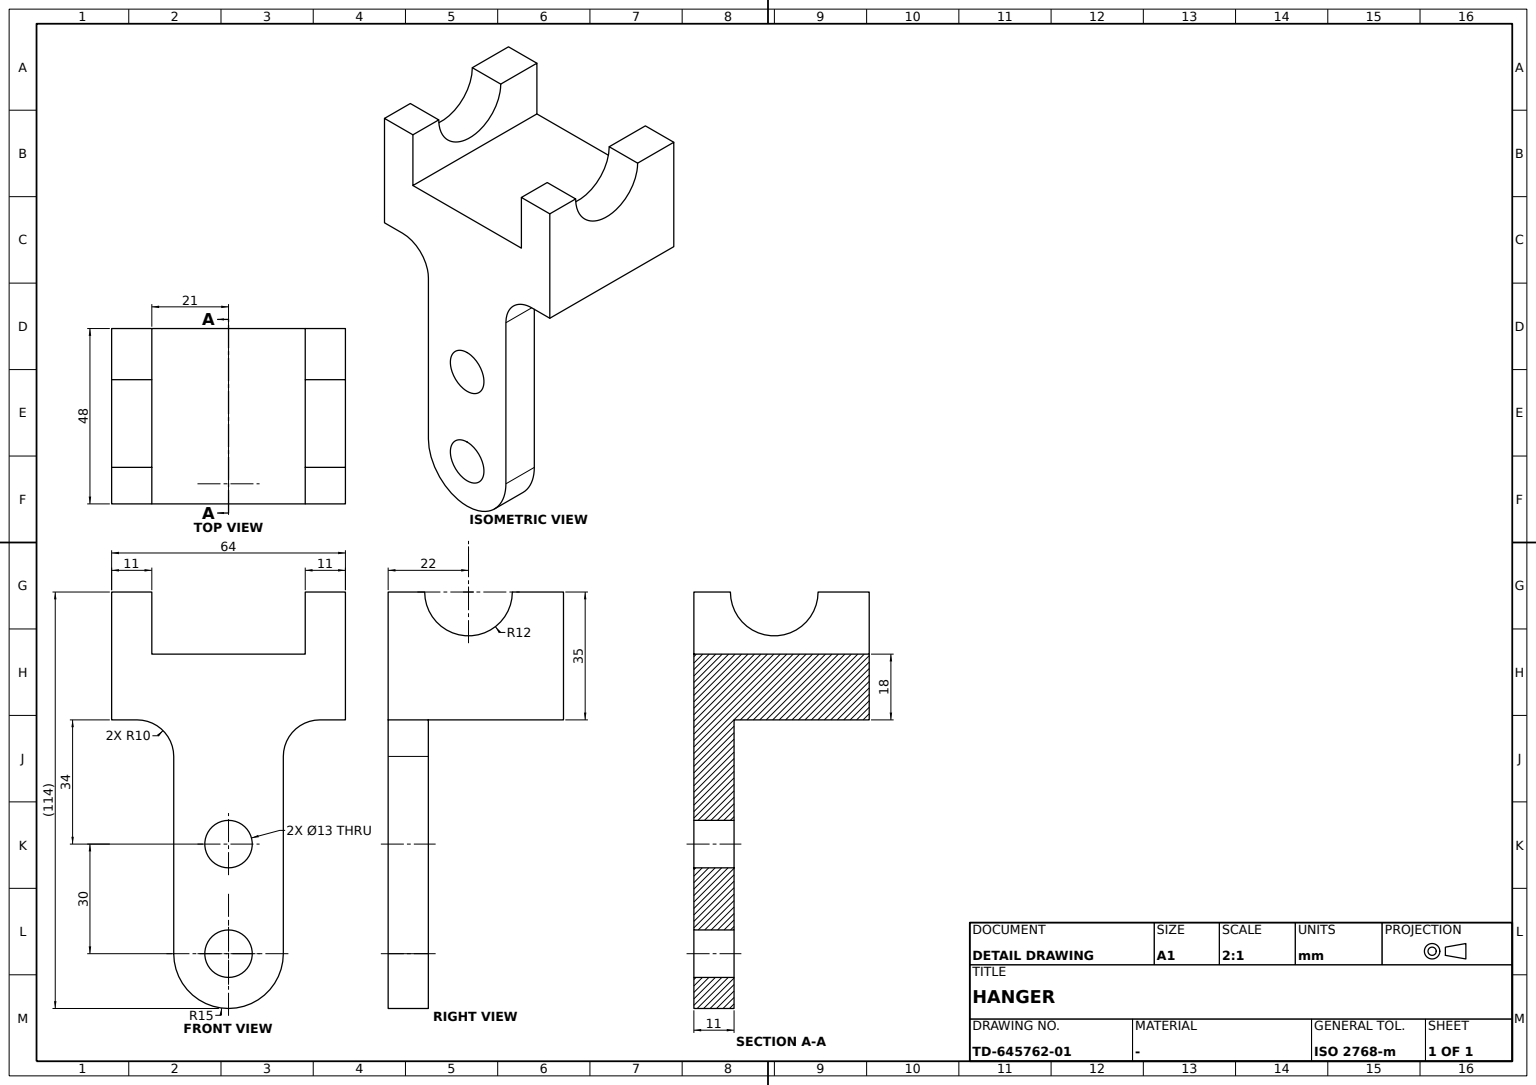
ISO-10303-21;
HEADER;
FILE_DESCRIPTION((''),'2;1');
FILE_NAME('','',(''),(''),'','','');
FILE_SCHEMA(('AUTOMOTIVE_DESIGN'));
ENDSEC;
DATA;
#1=APPLICATION_CONTEXT('');
#2=PRODUCT_CONTEXT('',#1,'mechanical');
#3=PRODUCT('','','',(#2));
#4=PRODUCT_DEFINITION_FORMATION('','',#3);
#5=PRODUCT_DEFINITION_CONTEXT('',#1,'design');
#6=PRODUCT_DEFINITION('','',#4,#5);
#7=PRODUCT_DEFINITION_SHAPE('','',#6);
#8=(LENGTH_UNIT()NAMED_UNIT(*)SI_UNIT(.MILLI.,.METRE.));
#9=(NAMED_UNIT(*)PLANE_ANGLE_UNIT()SI_UNIT($,.RADIAN.));
#10=(NAMED_UNIT(*)SI_UNIT($,.STERADIAN.)SOLID_ANGLE_UNIT());
#11=UNCERTAINTY_MEASURE_WITH_UNIT(LENGTH_MEASURE(0.005),#8,'distance_accuracy_value','');
#12=(GEOMETRIC_REPRESENTATION_CONTEXT(3)GLOBAL_UNCERTAINTY_ASSIGNED_CONTEXT((#11))GLOBAL_UNIT_ASSIGNED_CONTEXT((#8,#9,#10))REPRESENTATION_CONTEXT('',''));
#13=CARTESIAN_POINT('',(32.,48.,99.));
#14=VERTEX_POINT('',#13);
#15=CARTESIAN_POINT('',(32.,34.,99.));
#16=VERTEX_POINT('',#15);
#17=DIRECTION('',(0.,-1.,0.));
#18=VECTOR('',#17,1000.);
#19=LINE('',#13,#18);
#20=EDGE_CURVE('',#14,#16,#19,.T.);
#21=ORIENTED_EDGE('',*,*,#20,.F.);
#22=CARTESIAN_POINT('',(21.,48.,99.));
#23=VERTEX_POINT('',#22);
#24=DIRECTION('',(1.,0.,0.));
#25=VECTOR('',#24,1000.);
#26=LINE('',#22,#25);
#27=EDGE_CURVE('',#23,#14,#26,.T.);
#28=ORIENTED_EDGE('',*,*,#27,.F.);
#29=CARTESIAN_POINT('',(21.,34.,99.));
#30=VERTEX_POINT('',#29);
#31=LINE('',#22,#18);
#32=EDGE_CURVE('',#23,#30,#31,.T.);
#33=ORIENTED_EDGE('',*,*,#32,.T.);
#34=CARTESIAN_POINT('',(35.,34.,99.));
#35=LINE('',#34,#25);
#36=EDGE_CURVE('',#30,#16,#35,.T.);
#37=ORIENTED_EDGE('',*,*,#36,.T.);
#38=EDGE_LOOP('',(#21,#28,#33,#37));
#39=FACE_BOUND('',#38,.T.);
#40=DIRECTION('',(0.,0.,-1.));
#41=DIRECTION('',(-1.,0.,0.));
#42=AXIS2_PLACEMENT_3D('',#22,#40,#41);
#43=PLANE('',#42);
#44=ADVANCED_FACE('',(#39),#43,.F.);
#45=CARTESIAN_POINT('',(21.,48.,82.));
#46=VERTEX_POINT('',#45);
#47=CARTESIAN_POINT('',(21.,0.,82.));
#48=VERTEX_POINT('',#47);
#49=LINE('',#45,#18);
#50=EDGE_CURVE('',#46,#48,#49,.T.);
#51=ORIENTED_EDGE('',*,*,#50,.F.);
#52=CARTESIAN_POINT('',(-21.,48.,82.));
#53=VERTEX_POINT('',#52);
#54=LINE('',#52,#25);
#55=EDGE_CURVE('',#53,#46,#54,.T.);
#56=ORIENTED_EDGE('',*,*,#55,.F.);
#57=CARTESIAN_POINT('',(-21.,0.,82.));
#58=VERTEX_POINT('',#57);
#59=LINE('',#52,#18);
#60=EDGE_CURVE('',#53,#58,#59,.T.);
#61=ORIENTED_EDGE('',*,*,#60,.T.);
#62=LINE('',#57,#25);
#63=EDGE_CURVE('',#58,#48,#62,.T.);
#64=ORIENTED_EDGE('',*,*,#63,.T.);
#65=EDGE_LOOP('',(#51,#56,#61,#64));
#66=FACE_BOUND('',#65,.T.);
#67=AXIS2_PLACEMENT_3D('',#52,#40,#41);
#68=PLANE('',#67);
#69=ADVANCED_FACE('',(#66),#68,.F.);
#70=CARTESIAN_POINT('',(32.,10.,99.));
#71=VERTEX_POINT('',#70);
#72=CARTESIAN_POINT('',(32.,22.,99.));
#73=DIRECTION('',(0.,0.,1.));
#74=AXIS2_PLACEMENT_3D('',#72,#24,#73);
#75=CIRCLE('',#74,12.);
#76=EDGE_CURVE('',#71,#16,#75,.T.);
#77=ORIENTED_EDGE('',*,*,#76,.T.);
#78=ORIENTED_EDGE('',*,*,#36,.F.);
#79=CARTESIAN_POINT('',(21.,10.,99.));
#80=VERTEX_POINT('',#79);
#81=CARTESIAN_POINT('',(21.,22.,99.));
#82=AXIS2_PLACEMENT_3D('',#81,#41,#40);
#83=CIRCLE('',#82,12.);
#84=EDGE_CURVE('',#30,#80,#83,.T.);
#85=ORIENTED_EDGE('',*,*,#84,.T.);
#86=CARTESIAN_POINT('',(35.,10.,99.));
#87=VECTOR('',#41,1000.);
#88=LINE('',#86,#87);
#89=EDGE_CURVE('',#71,#80,#88,.T.);
#90=ORIENTED_EDGE('',*,*,#89,.F.);
#91=EDGE_LOOP('',(#77,#78,#85,#90));
#92=FACE_BOUND('',#91,.T.);
#93=CARTESIAN_POINT('',(35.,22.,99.));
#94=AXIS2_PLACEMENT_3D('',#93,#41,#73);
#95=CYLINDRICAL_SURFACE('',#94,12.);
#96=ADVANCED_FACE('',(#92),#95,.F.);
#97=CARTESIAN_POINT('',(-21.,10.,99.));
#98=VERTEX_POINT('',#97);
#99=CARTESIAN_POINT('',(-21.,0.,99.));
#100=VERTEX_POINT('',#99);
#101=CARTESIAN_POINT('',(-21.,48.,99.));
#102=LINE('',#101,#18);
#103=EDGE_CURVE('',#98,#100,#102,.T.);
#104=ORIENTED_EDGE('',*,*,#103,.F.);
#105=CARTESIAN_POINT('',(-32.,10.,99.));
#106=VERTEX_POINT('',#105);
#107=EDGE_CURVE('',#98,#106,#88,.T.);
#108=ORIENTED_EDGE('',*,*,#107,.T.);
#109=CARTESIAN_POINT('',(-32.,0.,99.));
#110=VERTEX_POINT('',#109);
#111=CARTESIAN_POINT('',(-32.,48.,99.));
#112=LINE('',#111,#18);
#113=EDGE_CURVE('',#106,#110,#112,.T.);
#114=ORIENTED_EDGE('',*,*,#113,.T.);
#115=LINE('',#109,#25);
#116=EDGE_CURVE('',#110,#100,#115,.T.);
#117=ORIENTED_EDGE('',*,*,#116,.T.);
#118=EDGE_LOOP('',(#104,#108,#114,#117));
#119=FACE_BOUND('',#118,.T.);
#120=AXIS2_PLACEMENT_3D('',#111,#40,#41);
#121=PLANE('',#120);
#122=ADVANCED_FACE('',(#119),#121,.F.);
#123=CARTESIAN_POINT('',(-21.,34.,99.));
#124=VERTEX_POINT('',#123);
#125=CARTESIAN_POINT('',(-21.,22.,99.));
#126=AXIS2_PLACEMENT_3D('',#125,#24,#73);
#127=CIRCLE('',#126,12.);
#128=EDGE_CURVE('',#98,#124,#127,.T.);
#129=ORIENTED_EDGE('',*,*,#128,.T.);
#130=CARTESIAN_POINT('',(-32.,34.,99.));
#131=VERTEX_POINT('',#130);
#132=EDGE_CURVE('',#131,#124,#35,.T.);
#133=ORIENTED_EDGE('',*,*,#132,.F.);
#134=CARTESIAN_POINT('',(-32.,22.,99.));
#135=AXIS2_PLACEMENT_3D('',#134,#41,#40);
#136=CIRCLE('',#135,12.);
#137=EDGE_CURVE('',#131,#106,#136,.T.);
#138=ORIENTED_EDGE('',*,*,#137,.T.);
#139=ORIENTED_EDGE('',*,*,#107,.F.);
#140=EDGE_LOOP('',(#129,#133,#138,#139));
#141=FACE_BOUND('',#140,.T.);
#142=ADVANCED_FACE('',(#141),#95,.F.);
#143=CARTESIAN_POINT('',(-25.,11.,64.));
#144=VERTEX_POINT('',#143);
#145=CARTESIAN_POINT('',(-25.,0.,64.));
#146=VERTEX_POINT('',#145);
#147=LINE('',#143,#18);
#148=EDGE_CURVE('',#144,#146,#147,.T.);
#149=ORIENTED_EDGE('',*,*,#148,.T.);
#150=CARTESIAN_POINT('',(-32.,0.,64.));
#151=VERTEX_POINT('',#150);
#152=CARTESIAN_POINT('',(32.,0.,64.));
#153=LINE('',#152,#87);
#154=EDGE_CURVE('',#146,#151,#153,.T.);
#155=ORIENTED_EDGE('',*,*,#154,.T.);
#156=CARTESIAN_POINT('',(-32.,48.,64.));
#157=VERTEX_POINT('',#156);
#158=LINE('',#156,#18);
#159=EDGE_CURVE('',#157,#151,#158,.T.);
#160=ORIENTED_EDGE('',*,*,#159,.F.);
#161=CARTESIAN_POINT('',(32.,48.,64.));
#162=VERTEX_POINT('',#161);
#163=LINE('',#161,#87);
#164=EDGE_CURVE('',#162,#157,#163,.T.);
#165=ORIENTED_EDGE('',*,*,#164,.F.);
#166=VERTEX_POINT('',#152);
#167=LINE('',#161,#18);
#168=EDGE_CURVE('',#162,#166,#167,.T.);
#169=ORIENTED_EDGE('',*,*,#168,.T.);
#170=CARTESIAN_POINT('',(25.,0.,64.));
#171=VERTEX_POINT('',#170);
#172=EDGE_CURVE('',#166,#171,#153,.T.);
#173=ORIENTED_EDGE('',*,*,#172,.T.);
#174=CARTESIAN_POINT('',(25.,11.,64.));
#175=VERTEX_POINT('',#174);
#176=LINE('',#174,#18);
#177=EDGE_CURVE('',#175,#171,#176,.T.);
#178=ORIENTED_EDGE('',*,*,#177,.F.);
#179=LINE('',#174,#87);
#180=EDGE_CURVE('',#175,#144,#179,.T.);
#181=ORIENTED_EDGE('',*,*,#180,.T.);
#182=EDGE_LOOP('',(#149,#155,#160,#165,#169,#173,#178,#181));
#183=FACE_BOUND('',#182,.T.);
#184=AXIS2_PLACEMENT_3D('',#161,#73,#24);
#185=PLANE('',#184);
#186=ADVANCED_FACE('',(#183),#185,.F.);
#187=CARTESIAN_POINT('',(0.,11.,36.5));
#188=VERTEX_POINT('',#187);
#189=CARTESIAN_POINT('',(0.,11.,23.5));
#190=VERTEX_POINT('',#189);
#191=CARTESIAN_POINT('',(0.,11.,30.));
#192=AXIS2_PLACEMENT_3D('',#191,#17,#24);
#193=CIRCLE('',#192,6.5);
#194=EDGE_CURVE('',#188,#190,#193,.T.);
#195=ORIENTED_EDGE('',*,*,#194,.F.);
#196=CARTESIAN_POINT('',(0.,0.,36.5));
#197=VERTEX_POINT('',#196);
#198=LINE('',#187,#18);
#199=EDGE_CURVE('',#197,#188,#198,.F.);
#200=ORIENTED_EDGE('',*,*,#199,.F.);
#201=CARTESIAN_POINT('',(0.,0.,23.5));
#202=VERTEX_POINT('',#201);
#203=CARTESIAN_POINT('',(0.,0.,30.));
#204=AXIS2_PLACEMENT_3D('',#203,#17,#24);
#205=CIRCLE('',#204,6.5);
#206=EDGE_CURVE('',#197,#202,#205,.T.);
#207=ORIENTED_EDGE('',*,*,#206,.T.);
#208=LINE('',#189,#18);
#209=EDGE_CURVE('',#190,#202,#208,.T.);
#210=ORIENTED_EDGE('',*,*,#209,.F.);
#211=EDGE_LOOP('',(#195,#200,#207,#210));
#212=FACE_BOUND('',#211,.T.);
#213=AXIS2_PLACEMENT_3D('',#191,#17,#40);
#214=CYLINDRICAL_SURFACE('',#213,6.5);
#215=ADVANCED_FACE('',(#212),#214,.F.);
#216=VERTEX_POINT('',#111);
#217=EDGE_CURVE('',#216,#131,#112,.T.);
#218=ORIENTED_EDGE('',*,*,#217,.T.);
#219=ORIENTED_EDGE('',*,*,#132,.T.);
#220=VERTEX_POINT('',#101);
#221=EDGE_CURVE('',#220,#124,#102,.T.);
#222=ORIENTED_EDGE('',*,*,#221,.F.);
#223=LINE('',#111,#25);
#224=EDGE_CURVE('',#216,#220,#223,.T.);
#225=ORIENTED_EDGE('',*,*,#224,.F.);
#226=EDGE_LOOP('',(#218,#219,#222,#225));
#227=FACE_BOUND('',#226,.T.);
#228=ADVANCED_FACE('',(#227),#121,.F.);
#229=ORIENTED_EDGE('',*,*,#55,.T.);
#230=VECTOR('',#73,1000.);
#231=LINE('',#45,#230);
#232=EDGE_CURVE('',#46,#23,#231,.T.);
#233=ORIENTED_EDGE('',*,*,#232,.T.);
#234=ORIENTED_EDGE('',*,*,#27,.T.);
#235=VECTOR('',#40,1000.);
#236=LINE('',#13,#235);
#237=EDGE_CURVE('',#14,#162,#236,.T.);
#238=ORIENTED_EDGE('',*,*,#237,.T.);
#239=ORIENTED_EDGE('',*,*,#164,.T.);
#240=LINE('',#156,#230);
#241=EDGE_CURVE('',#157,#216,#240,.T.);
#242=ORIENTED_EDGE('',*,*,#241,.T.);
#243=ORIENTED_EDGE('',*,*,#224,.T.);
#244=LINE('',#101,#235);
#245=EDGE_CURVE('',#220,#53,#244,.T.);
#246=ORIENTED_EDGE('',*,*,#245,.T.);
#247=EDGE_LOOP('',(#229,#233,#234,#238,#239,#242,#243,#246));
#248=FACE_BOUND('',#247,.T.);
#249=CARTESIAN_POINT('',(0.,48.,0.));
#250=AXIS2_PLACEMENT_3D('',#249,#17,#40);
#251=PLANE('',#250);
#252=ADVANCED_FACE('',(#248),#251,.F.);
#253=ORIENTED_EDGE('',*,*,#241,.F.);
#254=ORIENTED_EDGE('',*,*,#159,.T.);
#255=LINE('',#150,#230);
#256=EDGE_CURVE('',#151,#110,#255,.T.);
#257=ORIENTED_EDGE('',*,*,#256,.T.);
#258=ORIENTED_EDGE('',*,*,#113,.F.);
#259=ORIENTED_EDGE('',*,*,#137,.F.);
#260=ORIENTED_EDGE('',*,*,#217,.F.);
#261=EDGE_LOOP('',(#253,#254,#257,#258,#259,#260));
#262=FACE_BOUND('',#261,.T.);
#263=AXIS2_PLACEMENT_3D('',#156,#24,#40);
#264=PLANE('',#263);
#265=ADVANCED_FACE('',(#262),#264,.F.);
#266=CARTESIAN_POINT('',(15.,11.,0.));
#267=VERTEX_POINT('',#266);
#268=CARTESIAN_POINT('',(15.,11.,54.));
#269=VERTEX_POINT('',#268);
#270=LINE('',#266,#230);
#271=EDGE_CURVE('',#267,#269,#270,.T.);
#272=ORIENTED_EDGE('',*,*,#271,.T.);
#273=CARTESIAN_POINT('',(15.,0.,54.));
#274=VERTEX_POINT('',#273);
#275=LINE('',#268,#18);
#276=EDGE_CURVE('',#269,#274,#275,.T.);
#277=ORIENTED_EDGE('',*,*,#276,.T.);
#278=CARTESIAN_POINT('',(15.,0.,0.));
#279=VERTEX_POINT('',#278);
#280=LINE('',#278,#230);
#281=EDGE_CURVE('',#279,#274,#280,.T.);
#282=ORIENTED_EDGE('',*,*,#281,.F.);
#283=LINE('',#266,#18);
#284=EDGE_CURVE('',#267,#279,#283,.T.);
#285=ORIENTED_EDGE('',*,*,#284,.F.);
#286=EDGE_LOOP('',(#272,#277,#282,#285));
#287=FACE_BOUND('',#286,.T.);
#288=AXIS2_PLACEMENT_3D('',#266,#24,#40);
#289=PLANE('',#288);
#290=ADVANCED_FACE('',(#287),#289,.T.);
#291=EDGE_CURVE('',#190,#188,#193,.T.);
#292=ORIENTED_EDGE('',*,*,#291,.T.);
#293=ORIENTED_EDGE('',*,*,#194,.T.);
#294=EDGE_LOOP('',(#292,#293));
#295=FACE_BOUND('',#294,.T.);
#296=CARTESIAN_POINT('',(0.,11.,6.5));
#297=VERTEX_POINT('',#296);
#298=CARTESIAN_POINT('',(0.,11.,-6.5));
#299=VERTEX_POINT('',#298);
#300=CARTESIAN_POINT('',(0.,11.,0.));
#301=AXIS2_PLACEMENT_3D('',#300,#17,#24);
#302=CIRCLE('',#301,6.5);
#303=EDGE_CURVE('',#297,#299,#302,.T.);
#304=ORIENTED_EDGE('',*,*,#303,.T.);
#305=EDGE_CURVE('',#299,#297,#302,.T.);
#306=ORIENTED_EDGE('',*,*,#305,.T.);
#307=EDGE_LOOP('',(#304,#306));
#308=FACE_BOUND('',#307,.T.);
#309=CARTESIAN_POINT('',(0.,11.,-15.));
#310=VERTEX_POINT('',#309);
#311=CIRCLE('',#301,15.);
#312=EDGE_CURVE('',#310,#267,#311,.T.);
#313=ORIENTED_EDGE('',*,*,#312,.F.);
#314=CARTESIAN_POINT('',(-15.,11.,0.));
#315=VERTEX_POINT('',#314);
#316=EDGE_CURVE('',#315,#310,#311,.T.);
#317=ORIENTED_EDGE('',*,*,#316,.F.);
#318=CARTESIAN_POINT('',(-15.,11.,54.));
#319=VERTEX_POINT('',#318);
#320=LINE('',#318,#235);
#321=EDGE_CURVE('',#319,#315,#320,.T.);
#322=ORIENTED_EDGE('',*,*,#321,.F.);
#323=CARTESIAN_POINT('',(-25.,11.,54.));
#324=DIRECTION('',(0.,1.,0.));
#325=AXIS2_PLACEMENT_3D('',#323,#324,#24);
#326=CIRCLE('',#325,10.);
#327=EDGE_CURVE('',#144,#319,#326,.T.);
#328=ORIENTED_EDGE('',*,*,#327,.F.);
#329=ORIENTED_EDGE('',*,*,#180,.F.);
#330=CARTESIAN_POINT('',(25.,11.,54.));
#331=AXIS2_PLACEMENT_3D('',#330,#324,#24);
#332=CIRCLE('',#331,10.);
#333=EDGE_CURVE('',#269,#175,#332,.T.);
#334=ORIENTED_EDGE('',*,*,#333,.F.);
#335=ORIENTED_EDGE('',*,*,#271,.F.);
#336=EDGE_LOOP('',(#313,#317,#322,#328,#329,#334,#335));
#337=FACE_BOUND('',#336,.T.);
#338=AXIS2_PLACEMENT_3D('',#323,#324,#73);
#339=PLANE('',#338);
#340=ADVANCED_FACE('',(#295,#308,#337),#339,.T.);
#341=CARTESIAN_POINT('',(0.,0.,-15.));
#342=VERTEX_POINT('',#341);
#343=LINE('',#309,#18);
#344=EDGE_CURVE('',#310,#342,#343,.T.);
#345=ORIENTED_EDGE('',*,*,#344,.F.);
#346=ORIENTED_EDGE('',*,*,#312,.T.);
#347=ORIENTED_EDGE('',*,*,#284,.T.);
#348=CARTESIAN_POINT('',(0.,0.,0.));
#349=AXIS2_PLACEMENT_3D('',#348,#17,#24);
#350=CIRCLE('',#349,15.);
#351=EDGE_CURVE('',#342,#279,#350,.T.);
#352=ORIENTED_EDGE('',*,*,#351,.F.);
#353=EDGE_LOOP('',(#345,#346,#347,#352));
#354=FACE_BOUND('',#353,.T.);
#355=AXIS2_PLACEMENT_3D('',#300,#17,#40);
#356=CYLINDRICAL_SURFACE('',#355,15.);
#357=ADVANCED_FACE('',(#354),#356,.T.);
#358=CARTESIAN_POINT('',(0.,0.,6.5));
#359=VERTEX_POINT('',#358);
#360=CARTESIAN_POINT('',(0.,0.,-6.5));
#361=VERTEX_POINT('',#360);
#362=CIRCLE('',#349,6.5);
#363=EDGE_CURVE('',#359,#361,#362,.T.);
#364=ORIENTED_EDGE('',*,*,#363,.F.);
#365=EDGE_CURVE('',#361,#359,#362,.T.);
#366=ORIENTED_EDGE('',*,*,#365,.F.);
#367=EDGE_LOOP('',(#364,#366));
#368=FACE_BOUND('',#367,.T.);
#369=CARTESIAN_POINT('',(-15.,0.,54.));
#370=VERTEX_POINT('',#369);
#371=CARTESIAN_POINT('',(-25.,0.,54.));
#372=AXIS2_PLACEMENT_3D('',#371,#324,#24);
#373=CIRCLE('',#372,10.);
#374=EDGE_CURVE('',#146,#370,#373,.T.);
#375=ORIENTED_EDGE('',*,*,#374,.T.);
#376=CARTESIAN_POINT('',(-15.,0.,0.));
#377=VERTEX_POINT('',#376);
#378=LINE('',#369,#235);
#379=EDGE_CURVE('',#370,#377,#378,.T.);
#380=ORIENTED_EDGE('',*,*,#379,.T.);
#381=EDGE_CURVE('',#377,#342,#350,.T.);
#382=ORIENTED_EDGE('',*,*,#381,.T.);
#383=ORIENTED_EDGE('',*,*,#351,.T.);
#384=ORIENTED_EDGE('',*,*,#281,.T.);
#385=CARTESIAN_POINT('',(25.,0.,54.));
#386=AXIS2_PLACEMENT_3D('',#385,#324,#24);
#387=CIRCLE('',#386,10.);
#388=EDGE_CURVE('',#274,#171,#387,.T.);
#389=ORIENTED_EDGE('',*,*,#388,.T.);
#390=ORIENTED_EDGE('',*,*,#172,.F.);
#391=CARTESIAN_POINT('',(32.,0.,99.));
#392=VERTEX_POINT('',#391);
#393=LINE('',#391,#235);
#394=EDGE_CURVE('',#392,#166,#393,.T.);
#395=ORIENTED_EDGE('',*,*,#394,.F.);
#396=CARTESIAN_POINT('',(21.,0.,99.));
#397=VERTEX_POINT('',#396);
#398=LINE('',#396,#25);
#399=EDGE_CURVE('',#397,#392,#398,.T.);
#400=ORIENTED_EDGE('',*,*,#399,.F.);
#401=LINE('',#47,#230);
#402=EDGE_CURVE('',#48,#397,#401,.T.);
#403=ORIENTED_EDGE('',*,*,#402,.F.);
#404=ORIENTED_EDGE('',*,*,#63,.F.);
#405=LINE('',#99,#235);
#406=EDGE_CURVE('',#100,#58,#405,.T.);
#407=ORIENTED_EDGE('',*,*,#406,.F.);
#408=ORIENTED_EDGE('',*,*,#116,.F.);
#409=ORIENTED_EDGE('',*,*,#256,.F.);
#410=ORIENTED_EDGE('',*,*,#154,.F.);
#411=EDGE_LOOP('',(#375,#380,#382,#383,#384,#389,#390,#395,#400,#403,#404,#407,#408,#409,#410));
#412=FACE_BOUND('',#411,.T.);
#413=EDGE_CURVE('',#202,#197,#205,.T.);
#414=ORIENTED_EDGE('',*,*,#413,.F.);
#415=ORIENTED_EDGE('',*,*,#206,.F.);
#416=EDGE_LOOP('',(#414,#415));
#417=FACE_BOUND('',#416,.T.);
#418=AXIS2_PLACEMENT_3D('',#348,#17,#40);
#419=PLANE('',#418);
#420=ADVANCED_FACE('',(#368,#412,#417),#419,.T.);
#421=ORIENTED_EDGE('',*,*,#316,.T.);
#422=ORIENTED_EDGE('',*,*,#344,.T.);
#423=ORIENTED_EDGE('',*,*,#381,.F.);
#424=LINE('',#314,#18);
#425=EDGE_CURVE('',#315,#377,#424,.T.);
#426=ORIENTED_EDGE('',*,*,#425,.F.);
#427=EDGE_LOOP('',(#421,#422,#423,#426));
#428=FACE_BOUND('',#427,.T.);
#429=ADVANCED_FACE('',(#428),#356,.T.);
#430=LINE('',#298,#18);
#431=EDGE_CURVE('',#299,#361,#430,.T.);
#432=ORIENTED_EDGE('',*,*,#431,.T.);
#433=ORIENTED_EDGE('',*,*,#365,.T.);
#434=LINE('',#296,#18);
#435=EDGE_CURVE('',#359,#297,#434,.F.);
#436=ORIENTED_EDGE('',*,*,#435,.T.);
#437=ORIENTED_EDGE('',*,*,#305,.F.);
#438=EDGE_LOOP('',(#432,#433,#436,#437));
#439=FACE_BOUND('',#438,.T.);
#440=CYLINDRICAL_SURFACE('',#355,6.5);
#441=ADVANCED_FACE('',(#439),#440,.F.);
#442=ORIENTED_EDGE('',*,*,#89,.T.);
#443=EDGE_CURVE('',#80,#397,#31,.T.);
#444=ORIENTED_EDGE('',*,*,#443,.T.);
#445=ORIENTED_EDGE('',*,*,#399,.T.);
#446=EDGE_CURVE('',#71,#392,#19,.T.);
#447=ORIENTED_EDGE('',*,*,#446,.F.);
#448=EDGE_LOOP('',(#442,#444,#445,#447));
#449=FACE_BOUND('',#448,.T.);
#450=ADVANCED_FACE('',(#449),#43,.F.);
#451=ORIENTED_EDGE('',*,*,#425,.T.);
#452=ORIENTED_EDGE('',*,*,#379,.F.);
#453=LINE('',#318,#18);
#454=EDGE_CURVE('',#319,#370,#453,.T.);
#455=ORIENTED_EDGE('',*,*,#454,.F.);
#456=ORIENTED_EDGE('',*,*,#321,.T.);
#457=EDGE_LOOP('',(#451,#452,#455,#456));
#458=FACE_BOUND('',#457,.T.);
#459=AXIS2_PLACEMENT_3D('',#318,#41,#73);
#460=PLANE('',#459);
#461=ADVANCED_FACE('',(#458),#460,.T.);
#462=ORIENTED_EDGE('',*,*,#431,.F.);
#463=ORIENTED_EDGE('',*,*,#303,.F.);
#464=ORIENTED_EDGE('',*,*,#435,.F.);
#465=ORIENTED_EDGE('',*,*,#363,.T.);
#466=EDGE_LOOP('',(#462,#463,#464,#465));
#467=FACE_BOUND('',#466,.T.);
#468=ADVANCED_FACE('',(#467),#440,.F.);
#469=ORIENTED_EDGE('',*,*,#327,.T.);
#470=ORIENTED_EDGE('',*,*,#454,.T.);
#471=ORIENTED_EDGE('',*,*,#374,.F.);
#472=ORIENTED_EDGE('',*,*,#148,.F.);
#473=EDGE_LOOP('',(#469,#470,#471,#472));
#474=FACE_BOUND('',#473,.T.);
#475=AXIS2_PLACEMENT_3D('',#323,#17,#40);
#476=CYLINDRICAL_SURFACE('',#475,10.);
#477=ADVANCED_FACE('',(#474),#476,.F.);
#478=ORIENTED_EDGE('',*,*,#221,.T.);
#479=ORIENTED_EDGE('',*,*,#128,.F.);
#480=ORIENTED_EDGE('',*,*,#103,.T.);
#481=ORIENTED_EDGE('',*,*,#406,.T.);
#482=ORIENTED_EDGE('',*,*,#60,.F.);
#483=ORIENTED_EDGE('',*,*,#245,.F.);
#484=EDGE_LOOP('',(#478,#479,#480,#481,#482,#483));
#485=FACE_BOUND('',#484,.T.);
#486=AXIS2_PLACEMENT_3D('',#101,#41,#73);
#487=PLANE('',#486);
#488=ADVANCED_FACE('',(#485),#487,.F.);
#489=ORIENTED_EDGE('',*,*,#232,.F.);
#490=ORIENTED_EDGE('',*,*,#50,.T.);
#491=ORIENTED_EDGE('',*,*,#402,.T.);
#492=ORIENTED_EDGE('',*,*,#443,.F.);
#493=ORIENTED_EDGE('',*,*,#84,.F.);
#494=ORIENTED_EDGE('',*,*,#32,.F.);
#495=EDGE_LOOP('',(#489,#490,#491,#492,#493,#494));
#496=FACE_BOUND('',#495,.T.);
#497=AXIS2_PLACEMENT_3D('',#45,#24,#40);
#498=PLANE('',#497);
#499=ADVANCED_FACE('',(#496),#498,.F.);
#500=ORIENTED_EDGE('',*,*,#394,.T.);
#501=ORIENTED_EDGE('',*,*,#168,.F.);
#502=ORIENTED_EDGE('',*,*,#237,.F.);
#503=ORIENTED_EDGE('',*,*,#20,.T.);
#504=ORIENTED_EDGE('',*,*,#76,.F.);
#505=ORIENTED_EDGE('',*,*,#446,.T.);
#506=EDGE_LOOP('',(#500,#501,#502,#503,#504,#505));
#507=FACE_BOUND('',#506,.T.);
#508=AXIS2_PLACEMENT_3D('',#13,#41,#73);
#509=PLANE('',#508);
#510=ADVANCED_FACE('',(#507),#509,.F.);
#511=ORIENTED_EDGE('',*,*,#291,.F.);
#512=ORIENTED_EDGE('',*,*,#209,.T.);
#513=ORIENTED_EDGE('',*,*,#413,.T.);
#514=ORIENTED_EDGE('',*,*,#199,.T.);
#515=EDGE_LOOP('',(#511,#512,#513,#514));
#516=FACE_BOUND('',#515,.T.);
#517=ADVANCED_FACE('',(#516),#214,.F.);
#518=ORIENTED_EDGE('',*,*,#333,.T.);
#519=ORIENTED_EDGE('',*,*,#177,.T.);
#520=ORIENTED_EDGE('',*,*,#388,.F.);
#521=ORIENTED_EDGE('',*,*,#276,.F.);
#522=EDGE_LOOP('',(#518,#519,#520,#521));
#523=FACE_BOUND('',#522,.T.);
#524=AXIS2_PLACEMENT_3D('',#330,#17,#40);
#525=CYLINDRICAL_SURFACE('',#524,10.);
#526=ADVANCED_FACE('',(#523),#525,.F.);
#527=CLOSED_SHELL('',(#44,#69,#96,#122,#142,#186,#215,#228,#252,#265,#290,#340,#357,#420,#429,#441,#450,#461,#468,#477,#488,#499,#510,#517,#526));
#528=MANIFOLD_SOLID_BREP('',#527);
#529=ADVANCED_BREP_SHAPE_REPRESENTATION('',(#528),#12);
#530=SHAPE_DEFINITION_REPRESENTATION(#7,#529);
ENDSEC;
END-ISO-10303-21;
